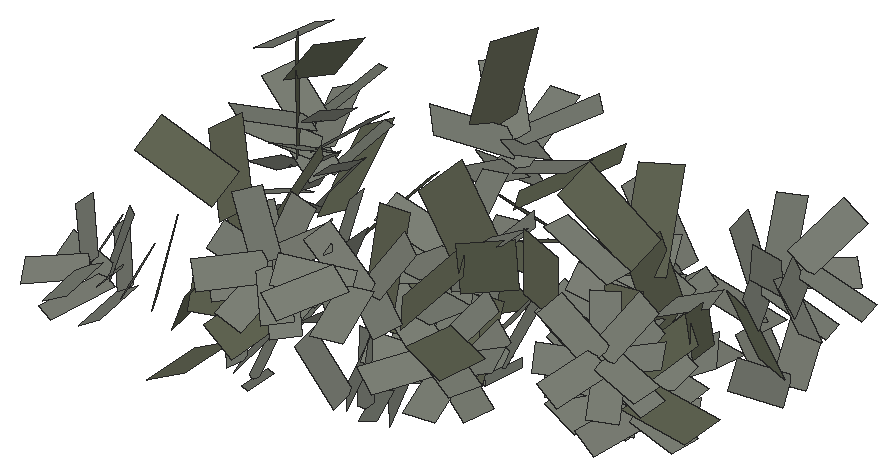
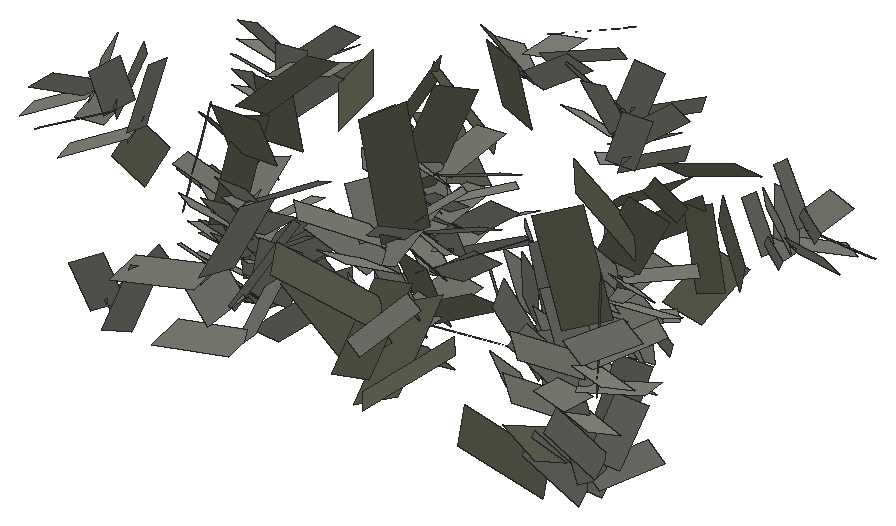
# SketchUp Ruby script. Lengths in inches.
U = 1.inch
M = Sketchup.active_model
def pt(a) = Geom::Point3d.new(a.map { |v| v * U })
def face(e, loops, mat)
  f = e.add_face(loops[0].map { |a| pt(a) })
  loops[1..].each { |l| e.add_face(l.map { |a| pt(a) }).erase! }
  f.material = f.back_material = mat if mat
  f
end
# faces: each face lists its corners as indices into pts; further lists are holes
def faces(e, pts, list, mat = nil) = list.each { |f| face(e, (f[0].is_a?(Array) ? f : [f]).map { |l| l.map { |i| pts[i] } }, mat) }
# xy, xz, yz: faces in a plane at the given z, y or x. An outline is a flat list of corners, or four numbers for a rectangle; further outlines are holes
def ring(l) = l.size == 4 ? [[l[0], l[1]], [l[2], l[1]], [l[2], l[3]], [l[0], l[3]]] : l.each_slice(2).to_a
def flat(e, list, mat, &to3) = list.each { |f| face(e, (f[0].is_a?(Array) ? f : [f]).map { |l| ring(l).map { |u, v| to3.(u, v) } }, mat) }
def xy(e, z, list, mat = nil) = flat(e, list, mat) { |x, y| [x, y, z] }
def xz(e, y, list, mat = nil) = flat(e, list, mat) { |x, z| [x, y, z] }
def yz(e, x, list, mat = nil) = flat(e, list, mat) { |y, z| [x, y, z] }
def lines(e, pts, list) = list.each { |a, b| e.add_line(pt(pts[a]), pt(pts[b])) }
# prism: a flat outline (further loops are holes) pulled along v
def prism(e, loops, v, mat = nil)
  f = face(e, loops, mat); d = Geom::Vector3d.new(v.map { |x| x * U })
  f.pushpull(f.normal.samedirection?(d) ? d.length : -d.length)
end
def box(e, o, s, mat = nil) = prism(e, [[o, [o[0] + s[0], o[1], o[2]], [o[0] + s[0], o[1] + s[1], o[2]], [o[0], o[1] + s[1], o[2]]]], [0, 0, s[2]], mat)
def at(x, y, z, deg = 0) = Geom::Transformation.translation(pt([x, y, z])) * Geom::Transformation.rotation(ORIGIN, Z_AXIS, deg.degrees)
def axes(o, x, y, z) = Geom::Transformation.new([*x, 0, *y, 0, *z, 0, *pt(o).to_a, 1])
def part(name) = M.definitions.add(name)
# library, detail: a bought-in or finely detailed component or shape, given as its bounding box
def library(name, o, s) = part(name).tap { |d| box(d.entities, o, s) }
def detail(e, o, s) = box(e.add_group.entities, o, s)
def put(e, d, t, mat = nil) = e.add_instance(d, t).tap { |i| i.material = mat if mat }
def group(e, t, mat = nil) = e.add_group.tap { |g| g.transformation = t; g.material = mat if mat }.entities
root = M.entities
M.materials.add("viburnumblaasdfas0df1w06d").color = [98, 102, 84]
M.materials.add("viburnumbladsadfasdfad0w122").color = [125, 129, 119]
c1 = part("Component\#315")
p = [[0.25,0,0],[2.05,0.01,0.35],[1.81,4.2,1.66],[0,4.19,1.3125]]
faces(c1.entities,p,[[0,1,2,3]],"viburnumbladsadfasdfad0w122")
c2 = part("viburnumblad2")
put(c2.entities,c1,axes([-19.23,-4.49,-32.18],[83.35428,0,0],[0,79.38502,0],[0,0,83.35428]))
c3 = part("Component\#314")
p = [[0.14,0,0],[2.58,0.05,0.25],[2.44,5.11,2.64],[0,5.05,2.39]]
faces(c3.entities,p,[[0,1,2,3]],"viburnumblaasdfas0df1w06d")
c4 = part("viburnumblad1\#2")
put(c4.entities,c3,axes([-37.25,6.23,19.31],[75.98784,0,0],[0,65.50676,0],[0,0,75.98784]))
put(root,c2,axes([2210.98,322.49,41],[-0.00995,0.00489,0.00397],[-0.00628,-0.00876,-0.0047],[0.00102,-0.00608,0.00892]))
put(root,c2,axes([2194.08,323.375,36.46],[-0.00855,-0.00051,-0.00592],[0.00282,-0.00961,-0.00317],[-0.00532,-0.00402,0.00702]))
put(root,c2,axes([2211.35,324.09,40.45],[-0.01153,-0.00217,-0.00126],[0.00257,-0.00998,-0.00587],[-0.00007,-0.00594,0.00905]))
put(root,c2,axes([2194.73,323.46,35.24],[-0.00848,0.00604,-0.00136],[-0.00422,-0.00741,-0.00622],[-0.00446,-0.0043,0.00739]))
put(root,c2,axes([2204.71,323.91,38.64],[-0.00593,0.00534,0.00783],[-0.0086,-0.00691,-0.00181],[0.00397,-0.00698,0.00778]))
put(root,c2,axes([2193.45,322.67,35.56],[-0.00345,0.00905,0.004],[-0.00908,-0.00113,-0.00507],[-0.00385,-0.00506,0.00725]))
put(root,c2,axes([2195.31,324.66,34.96],[-0.00729,-0.00007,-0.00611],[0.00282,-0.00961,-0.00317],[-0.00621,-0.00405,0.00634]))
put(root,c2,axes([2210.35,323.17,39.8],[-0.00254,0.00908,0.00688],[-0.01141,-0.00302,-0.00024],[0.00165,-0.00679,0.00837]))
put(root,c2,axes([2194.26,324.75,35.79],[-0.0036,-0.00676,-0.00701],[0.00718,-0.00608,0.00197],[-0.00593,-0.00439,0.00637]))
put(root,c2,axes([2205.21,324.92,39.49],[-0.00902,-0.00601,-0.00274],[0.00624,-0.00625,-0.00686],[0.00215,-0.00706,0.0084]))
put(root,c2,axes([2193.1,324.27,36.44],[0.00345,-0.00905,-0.004],[0.00788,-0.00012,0.00668],[-0.00594,-0.00519,0.00581]))
put(root,c2,axes([2204.74,325.5,38.12],[-0.01058,-0.00047,0.0036],[-0.00191,-0.00936,-0.00683],[0.00314,-0.00674,0.00835]))
put(root,c2,axes([2210.85,325.46,39.97],[-0.00572,-0.00664,-0.00612],[0.0099,-0.00571,-0.00294],[-0.00165,-0.00728,0.00803]))
put(root,c2,axes([2194.49,325.4375,34.85],[0.0036,-0.00945,-0.00418],[0.00709,-0.00011,0.00601],[-0.00594,-0.00519,0.00581]))
put(root,c2,axes([2193.57,323.57,34.57],[0.0036,0.00676,0.00701],[-0.00902,0.00536,-0.00055],[-0.00386,-0.00586,0.0067]))
put(root,c2,axes([2192.47,323.5625,35.54],[0.00855,0.00051,0.00592],[-0.00403,0.00835,0.00477],[-0.00448,-0.00623,0.00604]))
put(root,c2,axes([2203.74,324.75,37.72],[0.00218,0.00802,0.00747],[-0.00931,-0.0013,0.00412],[0.00416,-0.00766,0.007]))
put(root,c2,axes([2203.44,324.03,39.25],[0.00902,0.00601,0.00274],[-0.00554,0.00435,0.00868],[0.0036,-0.00837,0.00649]))
put(root,c2,axes([2203.78,325.8125,36.85],[-0.0062,0.00558,0.00817],[-0.00774,-0.00622,-0.00163],[0.00397,-0.00698,0.00778]))
put(root,c2,axes([2193.28,324.6,35.06],[0.00848,-0.00604,0.00136],[0.00312,0.00638,0.00815],[-0.00533,-0.00595,0.00568]))
put(root,c2,axes([2204.16,326.86,37.74],[-0.00866,-0.00577,-0.00263],[0.00674,-0.00675,-0.0074],[0.00215,-0.00706,0.0084]))
put(root,c4,axes([2199,328.07,31.14],[-0.01085,-0.00246,-0.00558],[0.00478,-0.01321,-0.00344],[-0.00438,-0.00417,0.00964]))
put(root,c2,axes([2209.78,324.26,38.95],[0.00611,0.00764,0.00552],[-0.01063,0.0043,0.00535],[0.00146,-0.00765,0.00773]))
put(root,c2,axes([2203.94,325.04,40.1],[0.00593,-0.00534,-0.00783],[0.00931,0.00502,0.00364],[0.00177,-0.00845,0.00711]))
put(root,c4,axes([2203.52,328.0625,35.08],[-0.00973,0.00003,0.00746],[-0.00524,-0.01136,-0.00678],[0.00594,-0.00739,0.00778]))
put(root,c2,axes([2204.17,326.14,39.05],[-0.00218,-0.00802,-0.00747],[0.01085,-0.00048,-0.00266],[0.00158,-0.00777,0.00788]))
put(root,c2,axes([2209.59,325.41,39.87],[0.01038,-0.0051,-0.00415],[0.00571,0.00633,0.00604],[-0.00053,-0.00802,0.00751]))
put(root,c2,axes([2193.96,324.66,33.93],[0.00821,0.00049,0.00568],[-0.00435,0.00902,0.00515],[-0.00448,-0.00623,0.00604]))
put(root,c4,axes([2196.98,327.89,32.46],[-0.00104,-0.01037,-0.00489],[0.01073,-0.00422,0.00645],[-0.0067,-0.00317,0.00766]))
put(root,c2,axes([2202.91,325.48,38.84],[0.01058,0.00047,-0.0036],[0.00255,0.00709,0.00842],[0.00261,-0.00869,0.00653]))
put(root,c4,axes([2195.3,326.74,32.91],[0.00672,-0.00928,0.00091],[0.00601,0.00561,0.01016],[-0.00772,-0.00461,0.00599]))
put(root,c2,axes([2202.7,325.81,37.39],[0.0079,0.00633,0.00186],[-0.00554,0.00435,0.00868],[0.00455,-0.00767,0.00675]))
put(root,c4,axes([2202.2,328.68,33.3125],[-0.0017,0.006,0.01056],[-0.01273,-0.00619,0.00147],[0.00521,-0.00927,0.00611]))
put(root,c2,axes([2223.12,328.97,37.56],[-0.00968,0.00131,0.00494],[-0.00342,-0.0096,-0.00398],[0.00374,-0.00505,0.00789]))
put(root,c4,axes([2209.18,326.8125,37.5],[0.01273,-0.00184,0.00122],[0.00029,0.0105,0.01027],[-0.0024,-0.00896,0.00784]))
put(root,c4,axes([2211.03,330.5625,35.06],[-0.00662,-0.01127,-0.00498],[0.01432,-0.00702,-0.0031],[-0.00011,-0.00548,0.01154]))
put(root,c4,axes([2198.26,327.98,39.05],[0.0023,0.0101,0.00657],[-0.0138,0.00343,-0.00044],[-0.0019,-0.0063,0.01035]))
put(root,c2,axes([2199.6,330.04,29.28],[-0.00404,-0.00727,-0.00631],[0.00772,-0.00559,0.00142],[-0.00472,-0.00433,0.00722]))
put(root,c2,axes([2222.91,330.49,37.07],[-0.00956,-0.00538,0.00002],[0.00454,-0.00801,-0.00608],[0.00277,-0.00525,0.00814]))
put(root,c4,axes([2209.58,328.98,36.74],[0.00746,-0.00961,-0.00443],[0.01187,0.00604,0.00656],[-0.00274,-0.0068,0.00947]))
put(root,c2,axes([2222.24,329.38,36.54],[-0.00413,0.00723,0.00696],[-0.00909,-0.00609,0.00092],[0.00444,-0.00548,0.00729]))
put(root,c2,axes([2211.08,330.11,32.95],[-0.00995,0.00489,0.00397],[-0.00607,-0.00954,-0.00338],[0.0019,-0.00477,0.00949]))
put(root,c2,axes([2222.8125,329.98,38.42],[-0.00385,-0.00891,-0.00491],[0.01001,-0.00205,-0.00401],[0.00209,-0.00597,0.00789]))
put(root,c2,axes([2198.58,329.54,30.09],[0.00345,-0.00905,-0.004],[0.00865,0.00062,0.00578],[-0.00475,-0.00515,0.0067]))
put(root,c2,axes([2221.84,328.45,37.71],[0.00385,0.00891,0.00491],[-0.00921,0.00054,0.0058],[0.00445,-0.00629,0.00669]))
put(root,c2,axes([2205.17,329.38,30.47],[0.00814,-0.00715,-0.0046],[0.00716,0.00216,0.00888],[-0.00455,-0.00881,0.00477]))
put(root,c2,axes([2206.23,330.47,30.01],[0.00034,-0.00733,-0.00907],[0.00978,-0.00348,0.00299],[-0.00497,-0.00808,0.00546]))
put(root,c2,axes([2201.07,330.99,33.14],[-0.0105,0.00104,-0.00371],[-0.00071,-0.0111,-0.00111],[-0.00379,-0.00081,0.01049]))
put(root,c2,axes([2200.22,329.98,34.15],[-0.00725,0.00846,-0.00094],[-0.008,-0.0072,-0.00303],[-0.00289,-0.00129,0.01072]))
put(root,c2,axes([2204.97,328.53,29.28],[0.00766,0.00322,0.00823],[-0.00853,0.00606,0.00527],[-0.00262,-0.00929,0.00521]))
put(root,c2,axes([2200.47,331.32,34.53],[-0.00759,-0.00699,-0.00431],[0.00673,-0.00866,0.00218],[-0.0047,-0.00111,0.01008]))
put(root,c2,axes([2211.33,331.63,32.21],[-0.01146,-0.00283,-0.00038],[0.00275,-0.01049,-0.00491],[0.00082,-0.00467,0.00968]))
put(root,c2,axes([2211,331.39,33.7],[-0.00626,-0.00889,-0.00451],[0.01001,-0.00557,-0.00285],[-0.00007,-0.00526,0.00943]))
put(root,c2,axes([2197.88,328.76,29.29],[0.00916,0.00124,0.00492],[-0.00387,0.00837,0.00487],[-0.00322,-0.0061,0.00681]))
put(root,c2,axes([2201.2,330.86,31.65],[-0.00696,0.00812,-0.0009],[-0.00864,-0.00777,-0.00327],[-0.00289,-0.00129,0.01072]))
put(root,c4,axes([2200.31,330.375,32.35],[0.01074,0.00549,0.00552],[-0.0086,0.00502,0.01173],[0.00238,-0.01127,0.00657]))
put(root,c2,axes([2198.55,329.81,28.67],[0.00892,-0.00552,0.00065],[0.00374,0.00694,0.00752],[-0.00413,-0.00589,0.00653]))
put(root,c2,axes([2221.53,329.47,38.57],[0.00968,-0.00131,-0.00494],[0.00422,0.00809,0.00577],[0.0028,-0.00722,0.00669]))
put(root,c2,axes([2222.01,331.54,36.73],[-0.00372,-0.00756,-0.00527],[0.01001,-0.00205,-0.00401],[0.00166,-0.0069,0.00731]))
put(root,c2,axes([2210.34,330.6,31.72],[-0.00261,0.00974,0.006],[-0.01123,-0.00353,0.00072],[0.00254,-0.00551,0.00899]))
put(root,c2,axes([2205.4,330.02,29.01],[0.01118,-0.00278,0.00257],[-0.00082,0.00655,0.0102],[-0.00357,-0.00931,0.00467]))
put(root,c2,axes([2221.32,330.16,35.86],[0.00369,0.00856,0.00471],[-0.00994,0.00059,0.00626],[0.00445,-0.00629,0.00669]))
put(root,c2,axes([2221.53,330.6875,37.75],[0.00413,-0.00723,-0.00696],[0.00908,0.00421,0.0008],[0.0021,-0.00679,0.00729]))
put(root,c4,axes([2197.78,329.25,37.22],[0.01004,0.00303,0.00636],[-0.00636,0.01197,0.00433],[-0.00443,-0.0059,0.0098]))
put(root,c2,axes([2221.18,329.625,37.13],[0.00956,0.00538,-0.00002],[-0.00388,0.00674,0.0082],[0.00377,-0.00701,0.00644]))
put(root,c2,axes([2206.29,331.43,29.09],[0.0085,-0.00746,-0.0048],[0.00645,0.00195,0.00799],[-0.00455,-0.00881,0.00477]))
put(root,c2,axes([2209.59,329.97,33.03],[0.00626,0.00889,0.00451],[-0.00973,0.00413,0.00504],[0.00235,-0.00645,0.00846]))
put(root,c2,axes([2200.15,330.29,32.62],[0.00024,0.01092,0.00238],[-0.01143,0.00081,-0.00255],[-0.00254,-0.00227,0.01065]))
put(root,c2,axes([2200.3,332.2,33.1],[-0.00024,-0.01092,-0.00238],[0.01005,-0.00131,0.00499],[-0.0051,-0.00202,0.00975]))
put(root,c2,axes([2210.73,332.9,31.61],[-0.00572,-0.00761,-0.00506],[0.01001,-0.00557,-0.00285],[-0.00075,-0.00619,0.00889]))
put(root,c4,axes([2213.08,333.87,37.12],[-0.00612,0.00474,0.0114],[-0.00511,-0.01476,0.0034],[0.01154,-0.00234,0.00716]))
put(root,c2,axes([2210.47,333.42,38.125],[-0.01249,0.00076,-0.00112],[-0.00058,-0.01239,-0.00197],[-0.00123,-0.0019,0.01236]))
put(root,c2,axes([2209.92,332.34,32.74],[0.00261,-0.00974,-0.006],[0.01057,0.00192,0.00135],[-0.00026,-0.0062,0.0089]))
put(root,c4,axes([2214.61,334.66,39.02],[-0.00769,-0.00672,0.00925],[0.00492,-0.01396,-0.00605],[0.01062,-0.00006,0.00878]))
put(root,c2,axes([2220.91,331.11,36.77],[0.01011,-0.00136,-0.00516],[0.0038,0.00729,0.00519],[0.0028,-0.00722,0.00669]))
put(root,c2,axes([2209.52,331.25,33.79],[0.00995,-0.00489,-0.00397],[0.00635,0.0081,0.00558],[0.00038,-0.00694,0.0084]))
put(root,c4,axes([2198.54,331.27,35.57],[0.00884,-0.00966,0.00214],[0.00883,0.00982,0.0079],[-0.00632,-0.00331,0.01118]))
put(root,c2,axes([2198.92,330.35,33.74],[0.00759,0.00699,0.00431],[-0.00767,0.00813,0.00032],[-0.00293,-0.00317,0.01031]))
put(root,c2,axes([2200.8125,334.17,32.66],[-0.0119,0.00385,-0.00772],[-0.00199,-0.01402,-0.00394],[-0.0084,-0.00214,0.01187]))
put(root,c2,axes([2199.17,331.6875,34.11],[0.00725,-0.00846,0.00094],[0.00707,0.00667,0.00553],[-0.00474,-0.00299,0.00967]))
put(root,c2,axes([2210.54,334.5625,35.17],[-0.01199,0.00073,-0.00108],[-0.00063,-0.01339,-0.00213],[-0.00123,-0.0019,0.01236]))
put(root,c2,axes([2210.17,333.42,36.4],[-0.00853,0.00907,0.00165],[-0.00968,-0.00877,-0.00184],[-0.00017,-0.0024,0.01233]))
put(root,c2,axes([2209.66,331.53,30.78],[0.00601,0.00853,0.00433],[-0.01051,0.00446,0.00545],[0.00235,-0.00645,0.00846]))
put(root,c2,axes([2199.24,331.22,32.46],[0.0105,-0.00104,0.00371],[-0.00021,0.00971,0.00332],[-0.00385,-0.00347,0.00991]))
put(root,c2,axes([2210.34,334.76,36.82],[-0.00913,-0.008,-0.00324],[0.00831,-0.00942,-0.00017],[-0.00232,-0.00227,0.01214]))
put(root,c2,axes([2199.86,331.1,31.24],[0.00793,0.00729,0.0045],[-0.0069,0.00732,0.00029],[-0.00293,-0.00317,0.01031]))
put(root,c2,axes([2199.99,332.24,31.625],[0.0071,-0.00744,-0.0001],[0.00707,0.00667,0.00553],[-0.00393,-0.00389,0.00972]))
put(root,c2,axes([2209.28,331.25,32.1875],[0.01146,0.00283,0.00038],[-0.00257,0.0094,0.00741],[0.00146,-0.00704,0.00821]))
put(root,c4,axes([2219.86,332.23,34.68],[0.0118,0.00221,-0.00034],[-0.00169,0.00933,0.00984],[0.00149,-0.00861,0.00716]))
put(root,c4,axes([2210.24,334.43,31.83],[-0.0066,0.01089,0.00527],[-0.0139,-0.00777,-0.00135],[0.00164,-0.00514,0.01268]))
put(root,c2,axes([2201.65,335.76,31.42],[-0.00909,-0.00693,-0.00924],[0.00664,-0.01276,0.00304],[-0.00946,-0.0023,0.01102]))
put(root,c2,axes([2209.15,332.625,37.76],[0.00042,0.01207,0.00346],[-0.01255,0.00034,0.00035],[0.00024,-0.00347,0.01207]))
put(root,c2,axes([2209.46,332.77,31.57],[0.01038,-0.0051,-0.00415],[0.00572,0.00729,0.00502],[0.00038,-0.00694,0.0084]))
put(root,c4,axes([2210.23,333.57,36.08],[0.00411,0.01355,0.00465],[-0.01078,-0.00135,0.01345],[0.01091,-0.00609,0.00813]))
put(root,c2,axes([2216.09,334.57,42.04],[-0.00224,-0.01174,-0.0016],[0.0107,-0.00091,-0.00829],[0.00736,-0.00274,0.0098]))
put(root,c2,axes([2209.61,334.73,38.4],[-0.00042,-0.01207,-0.00346],[0.01224,-0.00117,0.00258],[-0.0028,-0.00328,0.0118]))
put(root,c2,axes([2209.79,336.18,31.41],[-0.01244,-0.00019,-0.00567],[0.00199,-0.01294,-0.00394],[-0.00531,-0.00441,0.0118]))
put(root,c2,axes([2220,335.7,30.4],[-0.00968,0.00131,0.00494],[-0.00285,-0.01022,-0.00281],[0.00419,-0.00363,0.00837]))
put(root,c2,axes([2200.04,335.86,32.65],[-0.00095,-0.01366,-0.00535],[0.01077,-0.00429,0.00904],[-0.00996,-0.00334,0.01028]))
put(root,c2,axes([2209.29,333.64,34.8125],[0.00044,0.0126,0.00361],[-0.0113,0.00031,0.00032],[0.00024,-0.00347,0.01207]))
put(root,c4,axes([2220.07,336.08,32.36],[-0.00299,-0.01191,-0.00429],[0.01424,-0.00187,-0.0047],[0.00288,-0.00486,0.01046]))
put(root,c4,axes([2219.47,334.26,34.02],[0.00886,-0.00621,-0.00526],[0.00932,0.00889,0.00498],[0.00073,-0.00681,0.00878]))
put(root,c4,axes([2208.83,333.83,29.08],[0.01287,-0.00107,0.00071],[0.00034,0.01171,0.00907],[-0.00141,-0.0079,0.00892]))
put(root,c2,axes([2199.51,333.57,31.47],[0.00095,0.01366,0.00535],[-0.01286,0.00336,-0.00628],[-0.00706,-0.00428,0.01216]))
put(root,c2,axes([2208.7,333.4,36.22],[0.00913,0.008,0.00324],[-0.00792,0.00789,0.00285],[-0.00024,-0.00448,0.01173]))
put(root,c2,axes([2219.07,335.91,29.36],[-0.00449,0.00779,0.00619],[-0.00867,-0.00648,0.00177],[0.0049,-0.00408,0.00781]))
put(root,c2,axes([2218.16,337.7,31.47],[-0.01366,0.00095,0.00535],[-0.00336,-0.01286,-0.00628],[0.00428,-0.00706,0.01216]))
put(root,c2,axes([2208.76,335.09,36.74],[0.00853,-0.00907,-0.00165],[0.009,0.0076,0.00473],[-0.00239,-0.00435,0.01154]))
put(root,c2,axes([2208.29,333.93,38.03],[0.01249,-0.00076,0.00112],[0.00026,0.01157,0.0049],[-0.00133,-0.00485,0.01151]))
put(root,c2,axes([2209.91,337.84,30.23],[-0.00694,-0.00883,-0.00779],[0.00996,-0.00923,0.0016],[-0.00629,-0.00487,0.01112]))
put(root,c4,axes([2209.16,334.84,29.54],[0.0051,0.011,0.00655],[-0.01483,0.00551,0.0023],[-0.00067,-0.00681,0.01196]))
put(root,c2,axes([2219.64,336.8,31.15],[-0.00334,-0.0097,-0.00381],[0.01007,-0.00189,-0.00393],[0.0026,-0.00465,0.00851]))
put(root,c2,axes([2218.76,335.13,30.63],[0.00334,0.0097,0.00381],[-0.00915,0.00071,0.00588],[0.00496,-0.00497,0.00731]))
put(root,c2,axes([2208.7,335.27,30.4375],[-0.00263,0.0123,0.00535],[-0.01296,-0.00091,-0.00426],[-0.00348,-0.00589,0.01184]))
put(root,c4,axes([2218.99,336.17,38.87],[0.00217,0.0115,0.00524],[-0.01369,-0.00006,0.0058],[0.00451,-0.00566,0.01058]))
put(root,c2,axes([2208.62,337.44,31.55],[0.00263,-0.0123,-0.00535],[0.01173,-0.00054,0.007],[-0.00651,-0.00594,0.01045]))
put(root,c2,axes([2219.08,338.43,35.37],[-0.01126,-0.00309,0.00036],[0.00297,-0.01108,-0.00222],[0.00093,-0.00205,0.01147]))
put(root,c2,axes([2208.49,334.68,35.125],[0.01156,-0.00022,-0.00012],[0.00026,0.01157,0.0049],[0.00003,-0.0049,0.01157]))
put(root,c2,axes([2195.63,338.49,29.54],[-0.00877,-0.00751,-0.00615],[0.00336,-0.01013,0.00757],[-0.0091,0.00349,0.00872]))
put(root,c2,axes([2200.17,336.51,30.53],[0.00774,-0.01238,0.00167],[0.00805,0.00648,0.01066],[-0.00962,-0.00465,0.01009]))
put(root,c2,axes([2200.05,334.6,29.75],[0.00909,0.00693,0.00924],[-0.00802,0.01085,-0.00026],[-0.00757,-0.00532,0.01142]))
put(root,c2,axes([2218.625,338.34,33.81],[-0.00997,0.00542,0.0028],[-0.00605,-0.01063,-0.00096],[0.002,-0.00216,0.01131]))
put(root,c2,axes([2198.75,335.26,31.47],[0.0119,-0.00385,0.00772],[-0.0001,0.01309,0.00669],[-0.00863,-0.00547,0.01057]))
put(root,c2,axes([2218.09,336.52,28.61],[0.0032,0.00932,0.00366],[-0.00988,0.00076,0.00635],[0.00496,-0.00497,0.00731]))
put(root,c2,axes([2218.46,339.46,32.67],[-0.01081,-0.00296,0.00035],[0.0032,-0.01197,-0.0024],[0.00093,-0.00205,0.01147]))
put(root,c2,axes([2217.14,338.25,29.75],[-0.00693,0.00909,0.00924],[-0.01085,-0.00802,-0.00026],[0.00532,-0.00757,0.01142]))
put(root,c4,axes([2217.85,339.25,29.62],[-0.0084,0.0076,0.00599],[-0.00998,-0.01102,-0.00002],[0.00443,-0.00403,0.01133]))
put(root,c2,axes([2218.13,337.33,35.14],[-0.00283,0.01075,0.0036],[-0.01102,-0.00348,0.00171],[0.00265,-0.00298,0.01098]))
put(root,c2,axes([2218.31,337.32,30.42],[0.00449,-0.00779,-0.00619],[0.00881,0.00487,0.00016],[0.00266,-0.00553,0.00801]))
put(root,c2,axes([2218.4,336.23,31.39],[0.00968,-0.00131,-0.00494],[0.00378,0.00904,0.00475],[0.00337,-0.00599,0.00744]))
put(root,c2,axes([2216.47,336.9375,31.47],[0.00385,0.0119,0.00772],[-0.01309,-0.0001,0.00669],[0.00547,-0.00863,0.01057]))
put(root,c4,axes([2221.12,339.61,34.17],[-0.00543,0.00233,0.01137],[0.00034,-0.01453,0.00314],[0.0116,0.00141,0.00526]))
put(root,c2,axes([2218.01,336.16,29.9375],[0.0092,0.00594,-0.0008],[-0.00419,0.00749,0.00747],[0.00433,-0.00576,0.00715]))
put(root,c2,axes([2217.5625,339,32.66],[-0.00385,-0.0119,-0.00772],[0.01402,-0.00199,-0.00394],[0.00214,-0.0084,0.01187]))
put(root,c2,axes([2208.67,336.33,28.82],[0.00694,0.00883,0.00779],[-0.01027,0.00714,0.00105],[-0.0037,-0.00696,0.01117]))
put(root,c2,axes([2200.69,336.14,28.67],[0.01174,-0.00298,0.00601],[-0.0001,0.01309,0.00669],[-0.00729,-0.00586,0.01134]))
put(root,c2,axes([2218.42,339.57,34.23],[-0.00596,-0.00978,-0.00229],[0.01005,-0.00579,-0.00143],[0.00006,-0.0027,0.01137]))
put(root,c2,axes([2207.53,336.53,30.58],[0.01244,0.00019,0.00567],[-0.00322,0.01148,0.00668],[-0.00467,-0.00741,0.01049]))
put(root,c4,axes([2218.59,338.49,33.51],[0.00008,0.01316,0.00435],[-0.00745,-0.00443,0.01354],[0.01228,-0.00208,0.00607]))
put(root,c2,axes([2217.6,338.27,32.45],[-0.00295,0.01122,0.00376],[-0.00992,-0.00313,0.00154],[0.00265,-0.00298,0.01098]))
put(root,c2,axes([2224.84,340.2,37.51],[-0.00724,-0.00234,0.00954],[0.00229,-0.01023,-0.00078],[0.00905,0.00148,0.00724]))
put(root,c2,axes([2227.21,340.42,39.16],[-0.00693,-0.00224,0.00913],[0.00254,-0.01137,-0.00086],[0.00905,0.00148,0.00724]))
put(root,c2,axes([2208.29,338.05,29.61],[0.01065,-0.00857,0.00023],[0.00633,0.00812,0.0092],[-0.00584,-0.00699,0.01019]))
put(root,c2,axes([2217.64,337.56,29.41],[0.01011,-0.00136,-0.00516],[0.0034,0.00814,0.00428],[0.00337,-0.00599,0.00744]))
put(root,c4,axes([2222.4375,340.76,35.79],[-0.00364,-0.00823,0.00913],[0.00776,-0.0108,-0.00665],[0.01031,0.00314,0.00694]))
put(root,c2,axes([2225.9,339.78,38.375],[-0.00591,0.00652,0.00769],[-0.00251,-0.00882,0.00556],[0.0097,0.00126,0.00639]))
put(root,c2,axes([2217.97,339.32,35.76],[0.00283,-0.01075,-0.0036],[0.01134,0.00265,0.001],[-0.0001,-0.00373,0.01107]))
put(root,c2,axes([2217.33,337.88,33.8],[0.00596,0.00978,0.00229],[-0.00894,0.00456,0.00379],[0.00249,-0.00402,0.01069]))
put(root,c2,axes([2215.59,338.88,28.67],[0.00298,0.01174,0.00601],[-0.01309,-0.0001,0.00669],[0.00586,-0.00729,0.01134]))
put(root,c2,axes([2225.68,341.11,38.67],[-0.0039,-0.00969,0.00523],[0.00734,-0.00679,-0.00711],[0.00851,0.00087,0.00796]))
put(root,c4,axes([2217.27,337.61,37.12],[0.01321,0.00417,0.00061],[-0.00463,0.0136,0.00723],[0.00136,-0.00611,0.01237]))
put(root,c2,axes([2215.875,338.23,32.65],[0.01366,-0.00095,-0.00535],[0.00429,0.01077,0.00904],[0.00334,-0.00996,0.01028]))
put(root,c2,axes([2224.42,339.25,38.22],[-0.0023,0.01045,0.001],[-0.00575,-0.00222,0.00993],[0.00986,0.00159,0.00606]))
put(root,c2,axes([2215.22,338.36,30.53],[0.01238,0.00774,0.00167],[-0.00648,0.00805,0.01066],[0.00465,-0.00962,0.01009]))
put(root,c2,axes([2217.02,338.22,35.54],[0.01126,0.00309,-0.00036],[-0.00265,0.01026,0.00493],[0.00162,-0.00467,0.01059]))
put(root,c2,axes([2215.97,339.84,31.42],[0.00693,-0.00909,-0.00924],[0.01276,0.00664,0.00304],[0.0023,-0.00946,0.01102]))
put(root,c2,axes([2194.78,342.14,35.14],[-0.01197,-0.00238,-0.00293],[0.00194,-0.01232,0.00219],[-0.00304,0.00182,0.01144]))
put(root,c2,axes([2193.98,341.27,36.52],[-0.01008,0.00703,-0.00261],[-0.00714,-0.01028,-0.00011],[-0.00193,0.00159,0.01172]))
put(root,c4,axes([2206.62,343.5,29.26],[-0.01489,-0.00148,0.00524],[0.00198,-0.01828,0.00047],[0.00517,0.00094,0.01496]))
put(root,c2,axes([2207,342.54,37.82],[-0.01229,-0.00021,0.00042],[0.00023,-0.01336,0.00026],[0.00045,0.00027,0.01335]))
put(root,c2,axes([2216.93,339.39,34.34],[0.00997,-0.00542,-0.0028],[0.00614,0.00939,0.00366],[0.00055,-0.00455,0.01075]))
put(root,c2,axes([2206.8,341.49,39.26],[-0.00935,0.00927,0.0023],[-0.00914,-0.00973,0.00201],[0.00303,-0.00016,0.01302]))
put(root,c2,axes([2216.63,338.95,32.86],[0.01014,0.00329,-0.00138],[-0.00265,0.01026,0.00493],[0.00283,-0.00431,0.01049]))
put(root,c2,axes([2224.1,341.13,38.4],[0.00136,-0.01101,-0.00167],[0.00866,0.00241,-0.00886],[0.00838,-0.00019,0.00814]))
put(root,c4,axes([2193.41,342.96,38.15],[-0.00759,-0.01277,-0.00082],[0.01374,-0.0085,0.0061],[-0.0047,0.00228,0.01321]))
put(root,c2,axes([2226.56,341.45,40],[0.00142,-0.01147,-0.00174],[0.00801,0.00224,-0.0082],[0.00838,-0.00019,0.00814]))
put(root,c2,axes([2193.96,342.85,36.49],[-0.00685,-0.0104,-0.00154],[0.00967,-0.00694,0.00401],[-0.00399,0.00118,0.01121]))
put(root,c2,axes([2194.63,342.9,33.71],[-0.00587,-0.00963,-0.00252],[0.00967,-0.00694,0.00401],[-0.00471,0.00005,0.01098]))
put(root,c2,axes([2224.95,339.47,39.68],[0.0039,0.00969,-0.00523],[-0.00478,0.00655,0.00858],[0.00995,-0.00072,0.00609]))
put(root,c2,axes([2206.8,343.37,39.42],[-0.00935,-0.00954,0.00039],[0.00874,-0.00859,-0.00062],[0.00075,-0.0002,0.01334]))
put(root,c2,axes([2217.18,343.8,33.6],[-0.01234,0.00028,0.00961],[0.00075,-0.01555,0.00142],[0.00958,0.00158,0.01226]))
put(root,c4,axes([2192.77,341.79,34.28],[0.0095,-0.01111,0.00288],[0.00361,0.00703,0.01484],[-0.01096,-0.00785,0.00554]))
put(root,c2,axes([2193.72,340.96,34.9],[-0.00228,0.01232,-0.00076],[-0.01222,-0.00233,-0.0015],[-0.0013,0.00061,0.01189]))
put(root,c2,axes([2214.99,343.96,30.57],[-0.01223,0.0001,0.00757],[0.00075,-0.01555,0.00142],[0.00819,0.0016,0.01322]))
put(root,c2,axes([2215.65,342.88,32.24],[-0.00842,0.01125,0.00685],[-0.00786,-0.01092,0.00827],[0.01063,0.001,0.01143]))
put(root,c2,axes([2192.64,343.75,30.28],[-0.00935,-0.0054,-0.00582],[0.00328,-0.00946,0.00316],[-0.00651,0.0014,0.00804]))
put(root,c4,axes([2205.18,343.19,39.27],[-0.00382,-0.01538,-0.00062],[0.0121,-0.00355,0.01339],[-0.01131,0.00237,0.01086]))
put(root,c2,axes([2191.99,343.33,31.29],[-0.00946,0.00383,-0.00571],[-0.0036,-0.01015,-0.00104],[-0.00558,0.00147,0.00861]))
put(root,c2,axes([2191.2,344,32.39],[-0.00896,-0.00518,-0.00557],[0.00365,-0.01051,0.00351],[-0.00651,0.0014,0.00804]))
put(root,c2,axes([2224.91,340.97,39.73],[0.00591,-0.00652,-0.00769],[0.005,0.00963,-0.00433],[0.00875,-0.0011,0.00766]))
put(root,c2,axes([2223.21,343.16,29.28],[-0.00322,0.00766,0.00823],[-0.00606,-0.00853,0.00527],[0.00929,-0.00262,0.00521]))
put(root,c2,axes([2225.94,340.38,40.82],[0.00693,0.00224,-0.00913],[-0.00028,0.01139,0.00259],[0.0094,-0.00132,0.00681]))
put(root,c2,axes([2193.37,343.13,34.74],[0.00228,-0.01232,0.00076],[0.0106,0.00221,0.00397],[-0.00422,0.00003,0.01117]))
put(root,c2,axes([2206.11,343.67,37.96],[0,-0.01388,-0.00141],[0.01203,0.00003,-0.00025],[0.00028,-0.00135,0.01329]))
put(root,c2,axes([2215.68,345.09,32.22],[-0.00902,-0.01086,0.00673],[0.00875,-0.01029,-0.00487],[0.0085,0.00104,0.01308]))
put(root,c4,axes([2206.01,344.57,32.27],[-0.00484,-0.01365,0.00231],[0.016,-0.00575,-0.00049],[0.00117,0.00203,0.01447]))
put(root,c2,axes([2192.44,341.24,36.14],[0.00685,0.0104,0.00154],[-0.01034,0.00702,-0.00117],[-0.00153,-0.00054,0.01185]))
put(root,c2,axes([2193.51,341.22,33.32],[0.00658,0.00998,0.00148],[-0.01117,0.00758,-0.00127],[-0.00153,-0.00054,0.01185]))
put(root,c2,axes([2191.38,344.53,30.96],[-0.00321,-0.01115,-0.00217],[0.00909,-0.00398,0.00703],[-0.00713,0.00058,0.00765]))
put(root,c4,axes([2206.05,344.12,30.4],[-0.00859,0.01076,0.00042],[-0.01222,-0.00981,0.0027],[0.00229,0.0015,0.01233]))
put(root,c4,axes([2206.31,345.76,32.21],[-0.01366,0.00026,0.00163],[0.00037,-0.01516,0.00432],[0.00177,0.00434,0.01188]))
put(root,c2,axes([2205.125,341.72,39.53],[0.00935,0.00954,-0.00039],[-0.00905,0.00903,0.00388],[0.00303,-0.00246,0.01278]))
put(root,c2,axes([2215.87,342.7,34.58],[0.00042,0.01563,0.00009],[-0.01107,0.00024,0.01104],[0.01103,-0.00036,0.01108]))
put(root,c2,axes([2193.34,342.81,33.3],[0.01052,-0.00734,0.00272],[0.00582,0.00933,0.00265],[-0.0036,-0.00095,0.01134]))
put(root,c2,axes([2192.42,342.82,36.11],[0.01008,-0.00703,0.00261],[0.00646,0.01036,0.00294],[-0.0036,-0.00095,0.01134]))
put(root,c2,axes([2192.65,341.85,34.59],[0.01197,0.00238,0.00293],[-0.00273,0.01289,0.0007],[-0.00248,-0.00118,0.01162]))
put(root,c2,axes([2191.29,345.72,40],[-0.0088,0.00279,-0.00674],[-0.00068,-0.01083,-0.00359],[-0.00727,-0.00236,0.00851]))
put(root,c2,axes([2221.72,343.59,29.01],[0.00278,0.01118,0.00257],[-0.00655,-0.00082,0.0102],[0.00931,-0.00357,0.00467]))
put(root,c2,axes([2205.25,343.22,39.64],[0.00935,-0.00927,-0.0023],[0.00999,0.00977,0.00128],[0.00075,-0.00249,0.01311]))
put(root,c2,axes([2214.13,345.31,31.11],[-0.00044,-0.01632,-0.00009],[0.01207,-0.00029,-0.00723],[0.00803,-0.00029,0.01342]))
put(root,c2,axes([2216.32,345.4375,34.31],[-0.00042,-0.01563,-0.00009],[0.01341,-0.00032,-0.00803],[0.00803,-0.00029,0.01342]))
put(root,c4,axes([2194.65,343.4,28.36],[0.00673,-0.01108,0.00456],[0.01197,0.00933,0.00501],[-0.00603,0.0015,0.01157]))
put(root,c2,axes([2191.49,344.35,29.55],[0.00424,-0.01017,0.0024],[0.00881,0.00556,0.00708],[-0.00707,-0.00052,0.00766]))
put(root,c2,axes([2204.82,342.56,37.99],[0.0127,0.00018,-0.00182],[0.00025,0.01408,0.00318],[0.00189,-0.00295,0.0129]))
put(root,c4,axes([2193.68,342.22,30.28],[0.01245,-0.00088,0.00582],[0.00019,0.01586,0.00199],[-0.00575,-0.00142,0.01169]))
put(root,c4,axes([2204.97,344.03,34.73],[0.00753,-0.01256,0.00063],[0.01453,0.00876,0.0012],[-0.00121,0,0.01461]))
put(root,c2,axes([2205.74,345.79,35.11],[-0.01136,0.00626,-0.00167],[-0.00565,-0.00941,0.00229],[-0.00013,0.00352,0.01104]))
put(root,c2,axes([2190.1,344.72,31.73],[0.00442,-0.0106,0.0025],[0.00816,0.00515,0.00656],[-0.00707,-0.00052,0.00766]))
put(root,c2,axes([2222.35,343.36,30.47],[0.00715,0.00814,-0.0046],[-0.00216,0.00716,0.00888],[0.00881,-0.00455,0.00477]))
